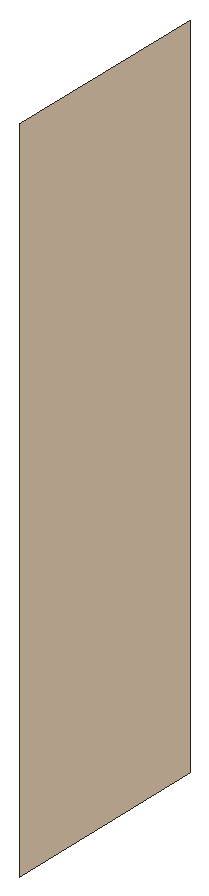
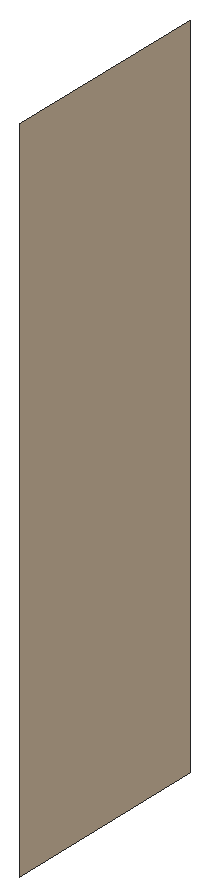
# SketchUp Ruby script. Lengths in inches.
U = 1.inch
M = Sketchup.active_model
def pt(a) = Geom::Point3d.new(a.map { |v| v * U })
def face(e, loops, mat)
  f = e.add_face(loops[0].map { |a| pt(a) })
  loops[1..].each { |l| e.add_face(l.map { |a| pt(a) }).erase! }
  f.material = f.back_material = mat if mat
  f
end
# faces: each face lists its corners as indices into pts; further lists are holes
def faces(e, pts, list, mat = nil) = list.each { |f| face(e, (f[0].is_a?(Array) ? f : [f]).map { |l| l.map { |i| pts[i] } }, mat) }
# xy, xz, yz: faces in a plane at the given z, y or x. An outline is a flat list of corners, or four numbers for a rectangle; further outlines are holes
def ring(l) = l.size == 4 ? [[l[0], l[1]], [l[2], l[1]], [l[2], l[3]], [l[0], l[3]]] : l.each_slice(2).to_a
def flat(e, list, mat, &to3) = list.each { |f| face(e, (f[0].is_a?(Array) ? f : [f]).map { |l| ring(l).map { |u, v| to3.(u, v) } }, mat) }
def xy(e, z, list, mat = nil) = flat(e, list, mat) { |x, y| [x, y, z] }
def xz(e, y, list, mat = nil) = flat(e, list, mat) { |x, z| [x, y, z] }
def yz(e, x, list, mat = nil) = flat(e, list, mat) { |y, z| [x, y, z] }
def lines(e, pts, list) = list.each { |a, b| e.add_line(pt(pts[a]), pt(pts[b])) }
# prism: a flat outline (further loops are holes) pulled along v
def prism(e, loops, v, mat = nil)
  f = face(e, loops, mat); d = Geom::Vector3d.new(v.map { |x| x * U })
  f.pushpull(f.normal.samedirection?(d) ? d.length : -d.length)
end
def box(e, o, s, mat = nil) = prism(e, [[o, [o[0] + s[0], o[1], o[2]], [o[0] + s[0], o[1] + s[1], o[2]], [o[0], o[1] + s[1], o[2]]]], [0, 0, s[2]], mat)
def at(x, y, z, deg = 0) = Geom::Transformation.translation(pt([x, y, z])) * Geom::Transformation.rotation(ORIGIN, Z_AXIS, deg.degrees)
def axes(o, x, y, z) = Geom::Transformation.new([*x, 0, *y, 0, *z, 0, *pt(o).to_a, 1])
def part(name) = M.definitions.add(name)
# library, detail: a bought-in or finely detailed component or shape, given as its bounding box
def library(name, o, s) = part(name).tap { |d| box(d.entities, o, s) }
def detail(e, o, s) = box(e.add_group.entities, o, s)
def put(e, d, t, mat = nil) = e.add_instance(d, t).tap { |i| i.material = mat if mat }
def group(e, t, mat = nil) = e.add_group.tap { |g| g.transformation = t; g.material = mat if mat }.entities
root = M.entities
M.materials.add("[0012_Bisque]1").color = [237, 212, 182]
yz(root,211.5,[[374.19,103.6875,403.76,197.75]],"[0012_Bisque]1")
